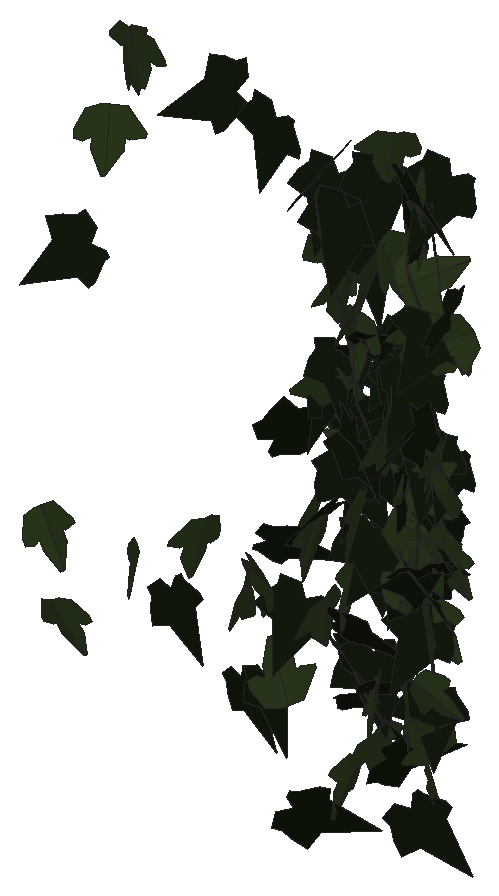
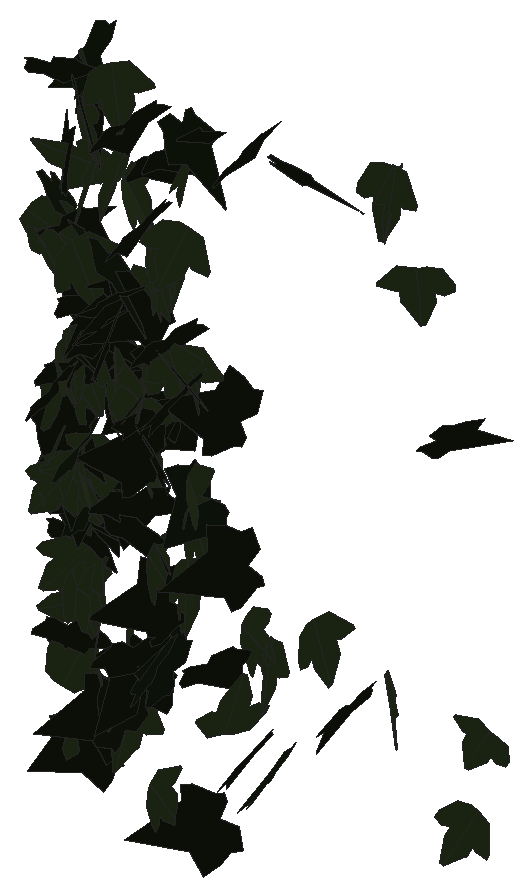
# SketchUp Ruby script. Lengths in inches.
U = 1.inch
M = Sketchup.active_model
def pt(a) = Geom::Point3d.new(a.map { |v| v * U })
def face(e, loops, mat)
  f = e.add_face(loops[0].map { |a| pt(a) })
  loops[1..].each { |l| e.add_face(l.map { |a| pt(a) }).erase! }
  f.material = f.back_material = mat if mat
  f
end
# faces: each face lists its corners as indices into pts; further lists are holes
def faces(e, pts, list, mat = nil) = list.each { |f| face(e, (f[0].is_a?(Array) ? f : [f]).map { |l| l.map { |i| pts[i] } }, mat) }
# xy, xz, yz: faces in a plane at the given z, y or x. An outline is a flat list of corners, or four numbers for a rectangle; further outlines are holes
def ring(l) = l.size == 4 ? [[l[0], l[1]], [l[2], l[1]], [l[2], l[3]], [l[0], l[3]]] : l.each_slice(2).to_a
def flat(e, list, mat, &to3) = list.each { |f| face(e, (f[0].is_a?(Array) ? f : [f]).map { |l| ring(l).map { |u, v| to3.(u, v) } }, mat) }
def xy(e, z, list, mat = nil) = flat(e, list, mat) { |x, y| [x, y, z] }
def xz(e, y, list, mat = nil) = flat(e, list, mat) { |x, z| [x, y, z] }
def yz(e, x, list, mat = nil) = flat(e, list, mat) { |y, z| [x, y, z] }
def lines(e, pts, list) = list.each { |a, b| e.add_line(pt(pts[a]), pt(pts[b])) }
# prism: a flat outline (further loops are holes) pulled along v
def prism(e, loops, v, mat = nil)
  f = face(e, loops, mat); d = Geom::Vector3d.new(v.map { |x| x * U })
  f.pushpull(f.normal.samedirection?(d) ? d.length : -d.length)
end
def box(e, o, s, mat = nil) = prism(e, [[o, [o[0] + s[0], o[1], o[2]], [o[0] + s[0], o[1] + s[1], o[2]], [o[0], o[1] + s[1], o[2]]]], [0, 0, s[2]], mat)
def at(x, y, z, deg = 0) = Geom::Transformation.translation(pt([x, y, z])) * Geom::Transformation.rotation(ORIGIN, Z_AXIS, deg.degrees)
def axes(o, x, y, z) = Geom::Transformation.new([*x, 0, *y, 0, *z, 0, *pt(o).to_a, 1])
def part(name) = M.definitions.add(name)
# library, detail: a bought-in or finely detailed component or shape, given as its bounding box
def library(name, o, s) = part(name).tap { |d| box(d.entities, o, s) }
def detail(e, o, s) = box(e.add_group.entities, o, s)
def put(e, d, t, mat = nil) = e.add_instance(d, t).tap { |i| i.material = mat if mat }
def group(e, t, mat = nil) = e.add_group.tap { |g| g.transformation = t; g.material = mat if mat }.entities
root = M.entities
M.materials.add("efeu1").color = [18, 25, 13]
M.materials.add("efeu2").color = [43, 57, 29]
c1 = part("ivyleaf_10")
p = [[0,0.5,-0.03],[-0.0625,2.02,-0.43],[-0.19,2.01,-0.46],[-0.54,1.05,-0.29],[-0.52,0.625,-0.18],[-0.83,0.76,-0.28],
  [-1.16,0.64,-0.33],[-1.15,0.33,-0.24],[-0.77,-0.39,0.02],[-0.3,-0.51,0.16],[0.04,-0.48,0.23],[-0.02,2.01,-0.4375],
  [-0.06,2.01,-0.43],[0.04,-0.49,0.23],[0.67,-0.49,0.14],[1.38,0.36,-0.2],[1.375,0.51,-0.24],[0.81,0.65,-0.19],
  [0.62,0.59,-0.15],[0.6,1.09,-0.28],[0.5,1.23,-0.31]]
faces(c1.entities,p,[[0,1,2,3,4,5,6,7,8,9,10],[11,12,0,13,14,15,16,17,18,19,20]],"efeu2")
c2 = part("ivyleaf_9")
p = [[1.54,2.16,1.25],[1.36,2.04,1.19],[-0.21,0.99,0.68],[-0.71,1.11,0.82],[-0.85,0.86,0.67],[-0.8,0.17,0.21],
  [-0.9,-0.01,0.1],[-0.67,-0.16,-0.02],[-0.08,-0.08,-0.05],[-0.03,-0.6,-0.4],[0.65,-0.88,-0.66],[0.83,-0.6,-0.49],
  [1.29,-0.42,-0.43],[1.8125,-0.07,-0.26],[1.21,0.44,0.15]]
faces(c2.entities,p,[[0,1,2,3,4,5,6,7,8,9,10,11,12,13,14]],"efeu1")
put(root,c1,axes([492,134.38,189.66],[0.60428,0.11496,0.41764],[0.41137,0.07226,-0.6151],[-0.1357,0.73099,-0.00488]))
put(root,c1,axes([492.57,134.4,186.96],[-0.68478,0.0523,-0.27904],[0.27876,-0.01407,-0.68674],[-0.05375,-0.73932,-0.00667]))
put(root,c2,axes([493.02,135.05,198.49],[-0.5303,-0.38728,0.42101],[-0.27163,-0.33475,-0.65008],[0.50343,-0.58857,0.09272]))
put(root,c1,axes([493.92,134.82,202.93],[0.67904,0.42585,-0.00571],[-0.00511,-0.00259,-0.80153],[-0.42586,0.67906,0.00052]))
put(root,c1,axes([494.72,135.07,205.65],[-0.81939,0.07604,0.0471],[-0.05104,-0.04109,-0.82165],[-0.07345,-0.81972,0.04556]))
put(root,c1,axes([494.78,134.73,205.48],[-0.28622,0.71836,0.28114],[-0.21645,0.21304,-0.7647],[-0.74043,-0.33997,0.11487]))
put(root,c1,axes([495.5,134.02,189.73],[0.45284,-0.57711,-0.21937],[-0.06683,0.22463,-0.72892],[0.61377,0.45025,0.08248]))
put(root,c2,axes([496.61,134.34,188.97],[0.29309,-0.66173,-0.24568],[-0.06104,0.24126,-0.72265],[0.70322,0.29673,0.03967]))
put(root,c1,axes([497.32,134.75,191.0625],[-0.13189,-0.74677,0.15508],[0.04,-0.16394,-0.7554],[0.76165,-0.12071,0.06652]))
put(root,c2,axes([497.99,135.32,205],[-0.74774,0.19425,0.27152],[-0.29552,-0.07525,-0.75999],[-0.15532,-0.79195,0.13881]))
put(root,c1,axes([499.03,134.5,189.75],[0.13459,-0.61433,-0.45784],[-0.011,0.46325,-0.62483],[0.76609,0.11458,0.07146]))
put(root,c2,axes([498.625,134.96,186.56],[0.43152,-0.617,-0.10754],[-0.03839,0.10429,-0.7524],[0.62512,0.43232,0.02803]))
put(root,c1,axes([499.73,134.52,190.15],[0.11039,0.09635,-0.77376],[-0.57861,0.53397,-0.01606],[0.52268,0.57076,0.14564]))
put(root,c2,axes([499.4,135.09,186.78],[0.25319,-0.71948,-0.02565],[-0.006,0.02508,-0.76273],[0.71991,0.25325,0.00266]))
put(root,c2,axes([499.5625,135.23,204.69],[-0.04078,-0.76036,0.31035],[0.00934,-0.31114,-0.76108],[0.82121,-0.03422,0.02407]))
put(root,c2,axes([500.33,135.53,189.43],[-0.3693,-0.6875,0.06625],[-0.02341,-0.06262,-0.78036],[0.69029,-0.36994,0.00897]))
put(root,c1,axes([500.52,134.42,187.125],[0.33572,0.73762,0.06695],[-0.05007,-0.05073,0.81006],[0.73896,-0.33856,0.02448]))
put(root,c2,axes([500.19,134.25,191.87],[0.63624,0.15608,0.45386],[0.43615,0.12651,-0.65492],[-0.20031,0.77122,0.01558]))
put(root,c2,axes([500.9,133.67,195.72],[0.15472,0.05272,0.79774],[0.70056,0.38255,-0.16115],[-0.38519,0.71692,0.02733]))
put(root,c2,axes([502.03,134.4375,204.4],[-0.41418,0.67967,-0.20007],[0.03283,-0.21309,-0.79186],[-0.70774,-0.40764,0.08036]))
put(root,c1,axes([501.67,134.46,192.78],[0.1436,-0.74511,0.25395],[0.128,-0.2326,-0.75486],[0.77672,0.17609,0.07745]))
put(root,c2,axes([501.79,133.78,193.09],[0.28373,0.5477,0.57038],[0.09518,0.55423,-0.61952],[-0.83167,0.25028,0.12369]))
put(root,c1,axes([501.64,135.11,201.47],[-0.74628,-0.1447,-0.26511],[0.27408,-0.02761,-0.75648],[0.12687,-0.79149,0.07486]))
put(root,c2,axes([501.3,134.03,183.79],[0.12138,0.24737,-0.79483],[0.36788,0.70461,0.27547],[0.74674,-0.38733,-0.00651]))
put(root,c1,axes([501.8,134.29,193.61],[0.28932,-0.71531,0.22891],[0.11948,-0.19835,-0.77081],[0.74148,0.31107,0.03489]))
put(root,c1,axes([502.07,134.47,197.42],[-0.66362,-0.42447,-0.01308],[0.00641,0.01425,-0.78771],[0.42462,-0.66359,-0.00855]))
put(root,c2,axes([501.61,135.26,196.87],[0.27569,-0.76338,-0.1447],[-0.01243,0.14918,-0.81073],[0.77687,0.27328,0.03838]))
put(root,c2,axes([501.96,135.02,197.46],[-0.64417,-0.10596,-0.44543],[0.45718,-0.10684,-0.63574],[0.02502,-0.77585,0.14838]))
put(root,c1,axes([502.46,134.69,197.36],[-0.62426,-0.13315,0.48153],[-0.44941,-0.22647,-0.60799],[0.26222,-0.70512,0.10434]))
put(root,c2,axes([502.07,134.84,203.92],[-0.27037,-0.76812,0.05811],[-0.01842,-0.05512,-0.81432],[0.7701,-0.271,0.00092]))
put(root,c1,axes([502.14,134.1,203.36],[-0.29158,0.7461,-0.09038],[0.01159,-0.08851,-0.82492],[-0.81115,-0.26946,0.0207]))
put(root,c1,axes([502.32,134.79,200.77],[-0.04468,-0.79721,-0.08124],[0.01166,0.08071,-0.79843],[0.80126,-0.04563,0.00709]))
put(root,c1,axes([502.32,133.92,190.69],[-0.03931,-0.75443,-0.23899],[0.03781,0.22827,-0.78515],[0.8509,-0.045,0.02384]))
put(root,c1,axes([502.2,135.34,184.85],[0.09983,-0.5844,0.42532],[0.15953,-0.40095,-0.58836],[0.70496,0.17349,0.07291]))
put(root,c2,axes([501.79,135.28,188.62],[0.45526,-0.5011,0.39711],[0.29012,-0.27251,-0.67648],[0.56976,0.53916,0.02715]))
put(root,c1,axes([502.34,134.6,200.3],[-0.61542,0.51955,-0.03984],[0.01528,-0.04133,-0.80168],[-0.56243,-0.56962,0.02182]))
put(root,c2,axes([502.2,134.99,198.2],[-0.04918,-0.78121,-0.10289],[0.01526,0.10213,-0.78271],[0.78781,-0.05075,0.00874]))
put(root,c2,axes([502.23,135.375,188.61],[0.44914,-0.63915,0.10465],[0.05155,-0.09167,-0.78111],[0.64561,0.45196,-0.01044]))
put(root,c1,axes([502.63,134.92,191.39],[0.16571,-0.57204,0.53633],[0.33846,-0.4423,-0.57633],[0.70734,0.34566,0.15012]))
put(root,c1,axes([502.93,134.78,199.53],[-0.76461,0.28303,-0.0868],[-0.03787,-0.2961,-0.73495],[-0.31643,-0.64847,0.29769]))
put(root,c1,axes([503.05,134.4,200.3125],[0.14495,-0.65789,-0.39377],[-0.08663,0.37005,-0.69829],[0.8152,0.1563,-0.00419]))
put(root,c2,axes([502.82,134.4,203.29],[-0.24262,-0.82107,0.00655],[-0.00215,-0.0062,-0.85616],[0.82109,-0.24263,-0.0003]))
put(root,c2,axes([502.98,134.92,194.88],[-0.63384,0.09369,-0.44304],[0.45836,-0.04215,-0.61772],[-0.10872,-0.72397,-0.02137]))
put(root,c2,axes([502.7,135.5,201.64],[0.15583,-0.79421,0.00354],[0.00064,-0.00348,-0.80935],[0.79422,0.15583,-0.00004]))
put(root,c1,axes([503.51,134.79,195.3],[0.34014,0.21951,0.68916],[-0.61586,-0.33842,0.39845],[0.43485,-0.65098,0.02525]))
put(root,c1,axes([503.24,134.48,197.0625],[-0.54364,0.49526,0.3469],[-0.25762,0.23316,-0.73441],[-0.59119,-0.55702,0.00103]))
put(root,c2,axes([502.83,134.46,195.32],[-0.1029,-0.5204,-0.6231],[0.18722,0.59595,-0.52864],[0.78995,-0.20903,0.04412]))
put(root,c2,axes([502.58,134.39,190.02],[0.74324,-0.12407,0.37068],[0.38827,-0.01,-0.72554],[0.12401,0.77495,0.04999]))
put(root,c2,axes([503.09,134.57,187.89],[0.58426,0.50724,0.17952],[0.08772,0.16483,-0.76846],[-0.57198,0.5434,0.06552]))
put(root,c2,axes([503.49,135.16,192.34],[-0.74075,-0.16588,-0.08521],[0.08616,0.01869,-0.73388],[0.18028,-0.6905,0.00061]))
put(root,c2,axes([503.07,135.24,188.79],[-0.1907,-0.68504,-0.37729],[0.08956,0.36666,-0.71101],[0.77692,-0.21042,-0.01064]))
put(root,c2,axes([502.68,135.1875,194.63],[0.60128,-0.26249,0.44766],[0.42357,-0.14758,-0.65547],[0.29981,0.73495,0.02826]))
put(root,c2,axes([502.9,134.71,198.89],[0.71,0.21754,0.32828],[0.30134,0.15818,-0.71773],[-0.28392,0.7119,0.05916]))
put(root,c1,axes([503.31,134.34,194.14],[0.31818,-0.66271,0.3683],[0.21299,-0.30521,-0.73318],[0.72764,0.37912,0.05356]))
put(root,c2,axes([503.09,134.68,196.35],[0.30081,-0.7274,0.2546],[0.08474,-0.24043,-0.78704],[0.766,0.31225,-0.01291]))
put(root,c1,axes([503.6,134.66,186.53],[-0.23672,-0.68474,-0.35407],[0.1053,0.33819,-0.72444],[0.76364,-0.25889,-0.00986]))
put(root,c2,axes([503.14,134.36,196.05],[-0.19372,-0.19084,-0.77693],[0.56733,0.53085,-0.27185],[0.56407,-0.59946,0.0066]))
put(root,c2,axes([503.4,134.875,193.03],[-0.28467,-0.66269,-0.37657],[0.16012,0.34101,-0.72116],[0.7452,-0.32642,0.0111]))
put(root,c2,axes([503.38,135.21,204.36],[-0.07186,-0.82224,-0.03527],[0.00553,0.03492,-0.82537],[0.82298,-0.07203,0.00247]))
put(root,c1,axes([503.85,135.15,205.55],[-0.51661,-0.52291,0.09233],[-0.05929,-0.0701,-0.73701],[0.56975,-0.48144,0.00703]))
put(root,c2,axes([503.18,135.53,186.5625],[0.08709,-0.39271,0.67056],[0.46642,-0.51328,-0.36118],[0.62155,0.4402,0.17708]))
put(root,c1,axes([503.82,134.4,201.97],[0.26579,-0.7063,0.29734],[0.09007,-0.28374,-0.75451],[0.76102,0.28026,-0.01455]))
put(root,c2,axes([504.37,134.6,199.75],[-0.44047,0.67683,0.17098],[-0.10974,0.13253,-0.80731],[-0.68942,-0.45353,0.01926]))
put(root,c2,axes([503.62,135.68,197.9375],[0.22959,-0.17133,-0.74563],[0.60187,-0.44014,0.28646],[-0.47231,-0.64417,0.00259]))
put(root,c2,axes([503.99,135.58,198.85],[-0.37818,-0.65843,0.26314],[0.00785,-0.3021,-0.74463],[0.70902,-0.34785,0.14861]))
put(root,c1,axes([503.75,134.44,188.34],[0.45085,-0.40375,0.54214],[0.40611,-0.35917,-0.6052],[0.54038,0.60678,0.00251]))
put(root,c2,axes([504.39,135.18,197.58],[-0.72555,-0.16253,0.08055],[-0.08058,-0.021,-0.71883],[0.17697,-0.67593,0.00297]))
put(root,c1,axes([503.67,134.9,196.83],[0.61805,-0.09915,0.50471],[0.5124,-0.10332,-0.6038],[0.15369,0.74319,-0.01661]))
put(root,c2,axes([503.93,135.57,198.14],[-0.0856,-0.79422,-0.03519],[-0.00204,0.03561,-0.7988],[0.795,-0.08542,-0.00583]))
put(root,c2,axes([503.85,134.77,197.32],[-0.07844,-0.31986,-0.74528],[0.437,0.6141,-0.30955],[0.68322,-0.42951,0.11243]))
put(root,c1,axes([504.39,134.29,196.67],[-0.0364,-0.81137,-0.1848],[0.03545,0.1833,-0.81175],[0.83139,-0.04334,0.02652]))
put(root,c1,axes([504.34,134.28,202.5],[-0.15516,0.73584,0.27848],[-0.0886,0.2566,-0.77911],[-0.84103,-0.16278,0.0307]))
put(root,c1,axes([504.54,134.03,197.61],[0.22745,-0.63084,-0.51206],[-0.13218,0.49593,-0.66969],[0.80168,0.26075,0.03486]))
put(root,c2,axes([504.21,134.98,198.73],[0.29177,-0.60977,-0.41938],[-0.0919,0.41745,-0.6709],[0.73433,0.29452,0.08266]))
put(root,c2,axes([504.29,134.44,186.28],[-0.01794,0.43454,-0.70073],[-0.00757,0.70078,0.43477],[0.8245,0.01589,-0.01126]))
put(root,c2,axes([504.5,133.55,195.79],[-0.23459,0.66513,-0.24781],[-0.0829,0.22559,0.72769],[0.75853,0.23036,0.00289]))
put(root,c1,axes([504.81,135.38,190.1875],[0.01336,-0.78462,0.19416],[0.04198,-0.19325,-0.78383],[0.80719,0.02304,0.03756]))
put(root,c1,axes([504.59,135.37,189.99],[0.06291,-0.49702,0.63173],[0.32789,-0.56268,-0.47535],[0.7339,0.294,0.15822]))
put(root,c1,axes([505.2,134.74,196.4],[-0.6034,-0.08641,0.40158],[-0.41453,-0.04399,-0.58782],[0.10385,-0.67773,-0.01305]))
put(root,c1,axes([504.98,135.2,199.88],[-0.27868,-0.71802,0.24819],[-0.05922,-0.24303,-0.76957],[0.75739,-0.28319,0.03115]))
put(root,c2,axes([505.42,133.65,195.49],[-0.1541,0.1223,-0.73999],[-0.76056,0.13621,0.17122],[0.17178,0.7128,0.09424]))
put(root,c2,axes([505.25,134.23,204.63],[0.36132,0.01288,-0.74343],[-0.77185,0.02797,-0.34733],[0.02147,0.78875,0.02445]))
put(root,c2,axes([504.98,134.9,198.54],[-0.4507,-0.6372,0.03949],[-0.03128,-0.02642,-0.79209],[0.68868,-0.4182,-0.01013]))
put(root,c1,axes([504.57,134.87,188.04],[0.1581,-0.24491,0.75063],[0.60169,-0.45833,-0.27627],[0.51127,0.61512,0.09301]))
put(root,c1,axes([505.39,134.4,203.48],[0.27394,-0.18598,-0.66498],[-0.43302,0.50364,-0.31777],[0.57421,0.46853,0.07762]))
put(root,c1,axes([505.1,133.85,191.98],[0.10105,0.52221,-0.42818],[0.0118,0.4145,0.54937],[0.71809,-0.0803,0.05123]))
put(root,c1,axes([504.76,135.2,193.39],[0.31073,-0.37169,0.60793],[0.44484,-0.41692,-0.48227],[0.55665,0.54066,0.04604]))
put(root,c1,axes([505.18,134.35,202.16],[-0.40019,0.57369,0.33146],[-0.16955,0.27789,-0.71005],[-0.6882,-0.40207,-0.01781]))
put(root,c1,axes([504.57,134.72,193.79],[-0.26968,-0.17728,-0.76835],[0.75537,0.17496,-0.30549],[0.22629,-0.79529,0.10407]))
put(root,c1,axes([505.66,134.05,204.52],[0.03387,0.09639,0.75877],[-0.73099,0.29045,-0.00965],[-0.31201,-0.67001,0.10498]))
put(root,c1,axes([505.03,134.84,195.42],[-0.02868,-0.03602,0.76583],[0.29635,-0.68439,-0.02452],[0.73903,0.27304,0.03955]))
put(root,c1,axes([505.36,135.07,185.28],[-0.4761,0.51474,-0.12812],[-0.08584,0.09413,0.70482],[0.56514,0.44794,-0.00088]))
put(root,c2,axes([505.74,134.16,203.94],[-0.30123,0.09245,-0.75622],[-0.74661,0.22543,0.30559],[0.26314,0.74545,0.00137]))
put(root,c1,axes([505.74,134.92,192.89],[-0.50765,-0.26171,0.54453],[-0.46213,-0.30459,-0.55784],[0.43138,-0.63428,0.0432]))
put(root,c2,axes([505.59,134,192.59],[0.11272,0.57869,-0.48397],[-0.15403,-0.44556,-0.6095],[-0.78707,0.17008,0.04997]))
put(root,c2,axes([505.85,133.97,197.03],[-0.05833,0.04213,0.77736],[-0.47733,0.60308,-0.06856],[-0.65261,-0.44487,-0.01933]))
put(root,c1,axes([505.03,135.13,190.84],[-0.62363,-0.20189,-0.46733],[0.51792,-0.07193,-0.60728],[0.12176,-0.72814,0.18957]))
put(root,c2,axes([505.78,134.93,194.7],[0.13613,0.17813,-0.6841],[-0.57827,-0.38793,-0.21596],[-0.4553,0.54597,0.06974]))
put(root,c1,axes([505.54,134.64,196.85],[0.60682,-0.18759,-0.47779],[-0.25501,0.53188,-0.5327],[0.44547,0.56001,0.3459]))
put(root,c2,axes([505.36,135.03,196.43],[-0.32783,-0.70465,-0.13201],[0.04197,0.12605,-0.77703],[0.71568,-0.33017,-0.01491]))
put(root,c1,axes([505.66,134.75,186.98],[-0.37518,-0.41366,-0.4349],[-0.29199,-0.31903,0.56179],[-0.56418,0.4402,-0.00154]))
put(root,c1,axes([505.49,134.73,192.84],[0.73935,-0.34011,-0.09704],[-0.07668,0.06666,-0.79446],[0.37309,0.68769,0.02902]))
put(root,c2,axes([505.02,135.14,194.09],[0.36316,-0.6093,0.3279],[0.18934,-0.26868,-0.70895],[0.66552,0.40892,0.02277]))
put(root,c2,axes([504.97,134.79,192.25],[0.40513,-0.55256,0.4427],[0.29469,-0.33217,-0.68429],[0.64378,0.49977,0.03465]))
put(root,c2,axes([505.73,134.03,192.98],[0.34433,0.67764,-0.19042],[-0.21182,-0.10709,-0.76737],[-0.7279,0.35171,0.13323]))
put(root,c2,axes([505.52,134.92,188.45],[-0.43181,-0.44494,-0.34723],[0.23833,0.25057,-0.62211],[0.55149,-0.45667,-0.00303]))
put(root,c2,axes([505.8125,134.38,191.125],[-0.72318,-0.32463,-0.10753],[0.11331,0.02043,-0.7734],[0.35007,-0.67724,0.02822]))
put(root,c2,axes([505.72,134.91,200.4],[-0.42893,-0.65321,0.1995],[-0.07616,-0.18837,-0.7805],[0.67874,-0.43394,0.03849]))
put(root,c1,axes([505.39,134.35,195.47],[0.29465,0.46968,0.57724],[0.24185,0.50973,-0.56307],[-0.74709,0.35025,0.04539]))
put(root,c1,axes([505.71,134.85,196.41],[0.25399,-0.74426,0.11013],[0.04832,-0.09986,-0.78629],[0.75081,0.2582,0.01335]))
put(root,c2,axes([505.51,135.7,195.86],[-0.03634,-0.73191,0.28257],[-0.0343,-0.28112,-0.73257],[0.78381,-0.04624,-0.01896]))
put(root,c2,axes([505.2,134.1,205.28],[0.61988,-0.55147,0.07936],[0.0593,-0.05299,-0.8278],[0.59833,0.57658,-0.00017]))
put(root,c2,axes([505.18,134.4,184.91],[-0.05533,-0.1495,-0.79723],[0.61382,0.51976,-0.14492],[0.57853,-0.56577,0.07752]))
put(root,c2,axes([505.97,134.54,201.92],[0.09295,-0.32107,0.72221],[-0.0771,0.69239,0.34213],[-0.82266,-0.10116,0.04954]))
put(root,c1,axes([506.26,134.46,195.52],[-0.45079,-0.03018,0.5383],[-0.55595,-0.05516,-0.43507],[0.06681,-0.66263,0.0117]))
put(root,c1,axes([505.64,135.16,192.92],[-0.61346,0.01742,-0.34884],[0.35968,-0.05618,-0.58958],[-0.047,-0.65726,0.04115]))
put(root,c1,axes([505.31,134.2,202.03],[0.40238,-0.04089,-0.73721],[0.7024,0.27994,0.36786],[0.22755,-0.79184,0.16811]))
put(root,c2,axes([505.98,134.96,205.15],[-0.68042,-0.47929,-0.10624],[0.16704,-0.05529,-0.82038],[0.46163,-0.68644,0.14026]))
put(root,c2,axes([506.375,134.42,201.12],[-0.58698,0.5525,0.01756],[-0.0135,0.01139,-0.80602],[-0.59683,-0.54365,0.00096]))
put(root,c1,axes([506.12,135.19,199.96],[0.6489,-0.17741,-0.27799],[-0.27817,0.07158,-0.65152],[0.20657,0.6537,-0.0041]))
put(root,c1,axes([505.55,134.44,189.01],[-0.34532,0.05622,-0.58472],[0.59715,-0.10192,-0.33763],[-0.12568,-0.63871,0.00241]))
put(root,c1,axes([505.88,134.94,193.48],[-0.20702,0.30555,0.60985],[0.26255,-0.53521,0.37268],[0.66411,0.30684,0.04277]))
put(root,c1,axes([506,134,191.55],[-0.49277,0.59078,-0.1232],[-0.00104,-0.14931,-0.77054],[-0.65074,-0.44713,0.09453]))
put(root,c1,axes([506.47,134.88,200.375],[0.40668,0.00544,-0.63346],[-0.65775,-0.00868,-0.39166],[-0.01106,0.71604,0.00007]))
put(root,c1,axes([505.7,134.91,193.5625],[-0.51909,0.31735,-0.50644],[0.44991,-0.25258,-0.59881],[-0.43777,-0.63589,-0.0149]))
